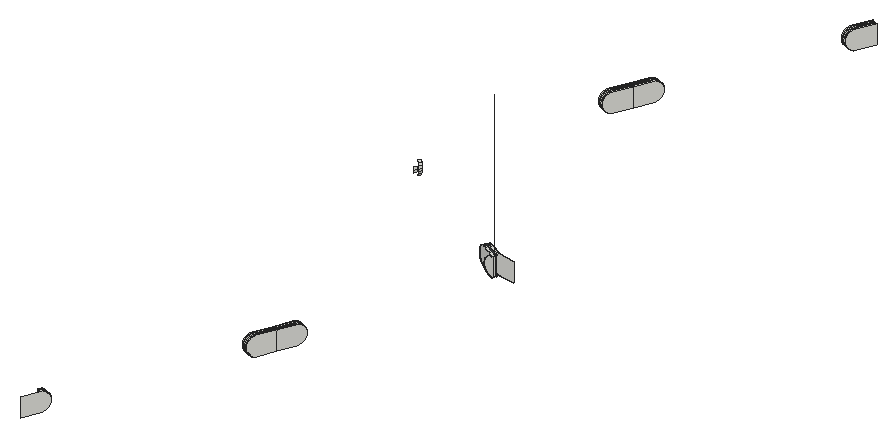
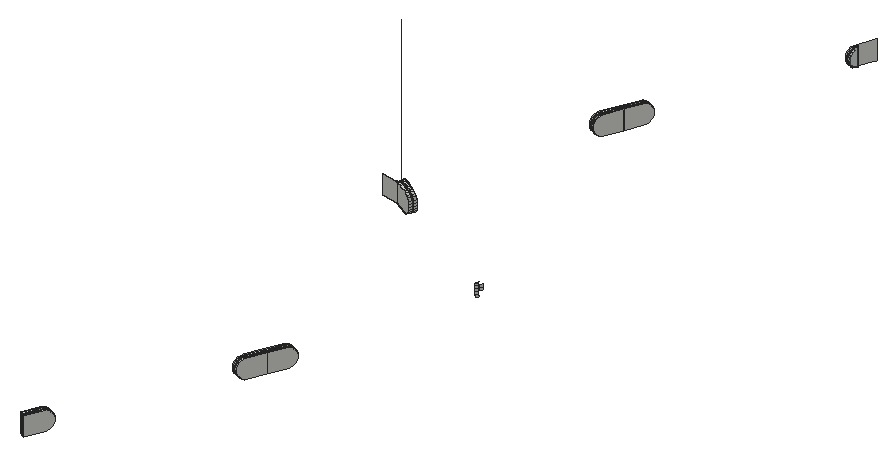
# SketchUp Ruby script. Lengths in inches.
U = 1.inch
M = Sketchup.active_model
def pt(a) = Geom::Point3d.new(a.map { |v| v * U })
def face(e, loops, mat)
  f = e.add_face(loops[0].map { |a| pt(a) })
  loops[1..].each { |l| e.add_face(l.map { |a| pt(a) }).erase! }
  f.material = f.back_material = mat if mat
  f
end
# faces: each face lists its corners as indices into pts; further lists are holes
def faces(e, pts, list, mat = nil) = list.each { |f| face(e, (f[0].is_a?(Array) ? f : [f]).map { |l| l.map { |i| pts[i] } }, mat) }
# xy, xz, yz: faces in a plane at the given z, y or x. An outline is a flat list of corners, or four numbers for a rectangle; further outlines are holes
def ring(l) = l.size == 4 ? [[l[0], l[1]], [l[2], l[1]], [l[2], l[3]], [l[0], l[3]]] : l.each_slice(2).to_a
def flat(e, list, mat, &to3) = list.each { |f| face(e, (f[0].is_a?(Array) ? f : [f]).map { |l| ring(l).map { |u, v| to3.(u, v) } }, mat) }
def xy(e, z, list, mat = nil) = flat(e, list, mat) { |x, y| [x, y, z] }
def xz(e, y, list, mat = nil) = flat(e, list, mat) { |x, z| [x, y, z] }
def yz(e, x, list, mat = nil) = flat(e, list, mat) { |y, z| [x, y, z] }
def lines(e, pts, list) = list.each { |a, b| e.add_line(pt(pts[a]), pt(pts[b])) }
# prism: a flat outline (further loops are holes) pulled along v
def prism(e, loops, v, mat = nil)
  f = face(e, loops, mat); d = Geom::Vector3d.new(v.map { |x| x * U })
  f.pushpull(f.normal.samedirection?(d) ? d.length : -d.length)
end
def box(e, o, s, mat = nil) = prism(e, [[o, [o[0] + s[0], o[1], o[2]], [o[0] + s[0], o[1] + s[1], o[2]], [o[0], o[1] + s[1], o[2]]]], [0, 0, s[2]], mat)
def at(x, y, z, deg = 0) = Geom::Transformation.translation(pt([x, y, z])) * Geom::Transformation.rotation(ORIGIN, Z_AXIS, deg.degrees)
def axes(o, x, y, z) = Geom::Transformation.new([*x, 0, *y, 0, *z, 0, *pt(o).to_a, 1])
def part(name) = M.definitions.add(name)
# library, detail: a bought-in or finely detailed component or shape, given as its bounding box
def library(name, o, s) = part(name).tap { |d| box(d.entities, o, s) }
def detail(e, o, s) = box(e.add_group.entities, o, s)
def put(e, d, t, mat = nil) = e.add_instance(d, t).tap { |i| i.material = mat if mat }
def group(e, t, mat = nil) = e.add_group.tap { |g| g.transformation = t; g.material = mat if mat }.entities
root = M.entities
M.materials.add("Glass_Safety_01").color = [204, 235, 244]
M.materials["Glass_Safety_01"].alpha = 0.1
xy(root,333,[[973.145,833.277,972.892,833.387,972.953,833.526,973.678,835.192,973.931,835.082],[972.711,833.465,972.459,833.576,973.241,835.37,973.496,835.268,972.772,833.605],[973.935,835.091,973.679,835.194,974.413,837.021,974.669,836.918],[973.496,835.268,973.241,835.37,973.245,835.38,973.497,835.27],[973.497,835.27,973.245,835.38,973.975,837.197,974.231,837.094],
  [980.412,857.229,978.702,858.205,978.839,858.444,980.548,857.469,980.545,857.462,980.493,857.47,980.474,857.338],[980.528,857.707,978.936,858.615,979.073,858.855,980.721,857.914,980.561,857.9375],[970.318,886.891,970.065,887.001,970.134,887.159,970.851,888.806,971.104,888.696],[969.884,887.079,969.632,887.189,970.418,888.994,970.671,888.884,969.953,887.238],[971.104,888.696,970.851,888.806,971.637,890.61,971.89,890.5],
  [970.671,888.884,970.418,888.994,971.204,890.799,971.457,890.689],[979.946,908.998,979.693,909.108,979.757,909.255,980.479,910.912,980.732,910.802],[979.513,909.186,979.26,909.296,980.046,911.101,980.299,910.991,979.577,909.334]])
xy(root,333.078,[[973.049,833.748,972.869,833.826,973.496,835.268,973.588,835.231,973.678,835.192],[973.679,835.194,973.588,835.231,973.497,835.27,974.084,836.729,974.267,836.655],[973.588,835.231,973.496,835.268,973.497,835.269,973.497,835.27],[980.548,857.469,979.181,858.249,979.278,858.42,980.63,857.649,980.611,857.652,980.597,857.554],[970.222,887.362,970.042,887.44,970.671,888.884,970.851,888.806],
  [970.851,888.806,970.671,888.884,971.299,890.328,971.48,890.249],[979.85,909.469,979.67,909.547,980.299,910.991,980.479,910.912]],"Glass_Safety_01")
xy(root,335.047,[[973.049,833.748,973.678,835.192,973.588,835.231,973.496,835.268,972.869,833.826],[973.679,835.194,974.267,836.655,974.084,836.729,973.497,835.27,973.588,835.231],[973.588,835.231,973.497,835.27,973.497,835.269,973.496,835.268],[980.548,857.469,980.597,857.554,980.611,857.652,980.63,857.649,979.278,858.42,979.181,858.249],[970.222,887.362,970.851,888.806,970.671,888.884,970.042,887.44],
  [970.851,888.806,971.48,890.249,971.299,890.328,970.671,888.884],[979.85,909.469,980.479,910.912,980.299,910.991,979.67,909.547]],"Glass_Safety_01")
xy(root,335.126,[[973.145,833.277,973.931,835.082,973.678,835.192,972.953,833.526,972.892,833.387],[972.711,833.465,972.772,833.605,973.496,835.268,973.241,835.37,972.459,833.576],[973.935,835.091,974.669,836.918,974.413,837.021,973.679,835.194],[973.496,835.268,973.497,835.27,973.245,835.38,973.241,835.37],[973.497,835.27,974.231,837.094,973.975,837.197,973.245,835.38],
  [980.412,857.229,980.474,857.338,980.493,857.47,980.545,857.462,980.548,857.469,978.839,858.444,978.702,858.205],[980.528,857.707,980.561,857.9375,980.721,857.914,979.073,858.855,978.936,858.615],[970.318,886.891,971.104,888.696,970.851,888.806,970.134,887.159,970.065,887.001],[969.884,887.079,969.953,887.238,970.671,888.884,970.418,888.994,969.632,887.189],[971.104,888.696,971.89,890.5,971.637,890.61,970.851,888.806],
  [970.671,888.884,971.457,890.689,971.204,890.799,970.418,888.994],[979.946,908.998,980.732,910.802,980.479,910.912,979.757,909.255,979.693,909.108],[979.513,909.186,979.577,909.334,980.299,910.991,980.046,911.101,979.26,909.296]])
p = [[963.767,811.746,335.126],[963.765,811.74,335.126],[963.765,811.74,333],[963.767,811.746,333],[963.77,811.753,333],[964.551,813.545,333],
  [964.661,813.797,333.036],[964.763,814.032,333.142],[964.851,814.234,333.311],[964.918,814.389,333.531],[964.961,814.486,333.787],[964.975,814.519,334.0625],
  [964.961,814.486,334.338],[964.918,814.389,334.594],[964.851,814.234,334.814],[964.763,814.032,334.983],[964.661,813.797,335.089],[964.551,813.545,335.126],
  [963.77,811.753,335.126],[964.298,813.655,333],[964.408,813.907,333.036],[964.118,813.733,333],[964.118,813.733,335.126],[964.227,813.986,335.089],
  [964.33,814.221,334.983],[964.418,814.423,334.814],[964.485,814.577,334.594],[964.528,814.675,334.338],[964.542,814.708,334.0625],[964.528,814.675,333.787],
  [964.485,814.577,333.531],[964.418,814.423,333.311],[964.33,814.221,333.142],[964.227,813.986,333.036],[964.298,813.655,335.126],[964.51,814.142,333.142],
  [964.598,814.344,333.311],[964.666,814.499,333.531],[964.708,814.596,333.787],[964.723,814.629,334.0625],[964.708,814.596,334.338],[964.666,814.499,334.594],
  [964.598,814.344,334.814],[964.51,814.142,334.983],[964.408,813.907,335.089],[973.931,835.082,335.126],[973.145,833.277,335.126],[973.035,833.025,335.089],
  [972.932,832.79,334.983],[972.844,832.588,334.814],[972.777,832.433,334.594],[972.735,832.335,334.338],[972.72,832.302,334.0625],[972.735,832.335,333.787],
  [972.777,832.433,333.531],[972.844,832.588,333.311],[972.932,832.79,333.142],[973.035,833.025,333.036],[973.145,833.277,333],[973.931,835.082,333],
  [972.892,833.387,335.126],[972.953,833.526,335.126],[972.953,833.526,333],[972.892,833.387,333],[972.782,833.135,333.036],[972.68,832.9,333.142],
  [972.592,832.698,333.311],[972.524,832.543,333.531],[972.482,832.446,333.787],[972.467,832.412,334.0625],[972.482,832.446,334.338],[972.524,832.543,334.594],
  [972.592,832.698,334.814],[972.68,832.9,334.983],[972.782,833.135,335.089],[972.711,833.465,333],[972.772,833.605,333],[973.496,835.268,333],
  [973.496,835.268,333.078],[973.496,835.268,335.047],[973.496,835.268,335.126],[972.772,833.605,335.126],[972.711,833.465,335.126],[972.602,833.213,335.089],
  [972.499,832.978,334.983],[972.411,832.776,334.814],[972.344,832.621,334.594],[972.301,832.524,334.338],[972.287,832.491,334.0625],[972.301,832.524,333.787],
  [972.344,832.621,333.531],[972.411,832.776,333.311],[972.499,832.978,333.142],[972.602,833.213,333.036],[972.459,833.576,335.126],[973.241,835.37,335.126],
  [973.241,835.37,333],[972.459,833.576,333],[972.349,833.323,333.036],[972.247,833.088,333.142],[972.159,832.886,333.311],[972.091,832.732,333.531],
  [972.049,832.634,333.787],[972.034,832.601,334.0625],[972.049,832.634,334.338],[972.091,832.732,334.594],[972.159,832.886,334.814],[972.247,833.088,334.983],
  [972.349,833.323,335.089],[973.678,835.192,333],[973.678,835.192,335.126],[973.678,835.192,335.047],[973.049,833.748,335.047],[973.049,833.748,333.078],
  [973.678,835.192,333.078],[973.679,835.194,333.078],[973.679,835.194,333],[973.935,835.091,333],[973.935,835.091,335.126],[973.679,835.194,335.126],
  [973.679,835.194,335.047],[974.669,836.918,335.126],[974.669,836.918,333],[974.772,837.173,333.036],[974.867,837.411,333.142],[974.95,837.615,333.311],
  [975.013,837.772,333.531],[975.052,837.87,333.787],[975.066,837.904,334.0625],[975.052,837.87,334.338],[975.013,837.772,334.594],[974.95,837.615,334.814],
  [974.867,837.411,334.983],[974.772,837.173,335.089],[974.413,837.021,335.126],[974.413,837.021,333],[974.267,836.655,333.078],[974.267,836.655,335.047],
  [973.497,835.27,333.078],[973.497,835.27,333],[973.245,835.38,333],[973.245,835.38,335.126],[973.497,835.27,335.126],[973.497,835.27,335.047],
  [974.231,837.094,333],[974.333,837.349,333.036],[974.429,837.587,333.142],[974.511,837.791,333.311],[974.574,837.948,333.531],[974.614,838.047,333.787],
  [974.627,838.08,334.0625],[974.614,838.047,334.338],[974.574,837.948,334.594],[974.511,837.791,334.814],[974.429,837.587,334.983],[974.333,837.349,335.089],
  [974.231,837.094,335.126],[973.243,835.375,333],[973.243,835.375,335.126],[973.975,837.197,335.126],[974.078,837.452,335.089],[974.173,837.69,334.983],
  [974.256,837.894,334.814],[974.319,838.051,334.594],[974.358,838.149,334.338],[974.372,838.183,334.0625],[974.358,838.149,333.787],[974.319,838.051,333.531],
  [974.256,837.894,333.311],[974.173,837.69,333.142],[974.078,837.452,333.036],[973.975,837.197,333],[974.516,837.276,333.036],[974.612,837.514,333.142],
  [974.694,837.718,333.311],[974.757,837.875,333.531],[974.797,837.973,333.787],[974.81,838.007,334.0625],[974.797,837.973,334.338],[974.757,837.875,334.594],
  [974.694,837.718,334.814],[974.612,837.514,334.983],[974.516,837.276,335.089],[980.412,857.229,335.126],[978.702,858.205,335.126],[978.463,858.341,335.089],
  [978.24,858.468,334.983],[978.049,858.578,334.814],[977.902,858.661,334.594],[977.81,858.714,334.338],[977.779,858.732,334.0625],[977.81,858.714,333.787],
  [977.902,858.661,333.531],[978.049,858.578,333.311],[978.24,858.468,333.142],[978.463,858.341,333.036],[978.702,858.205,333],[980.412,857.229,333],
  [980.453,857.197,333],[980.543,857.184,333],[980.543,857.184,335.126],[980.453,857.197,335.126],[980.181,857.237,335.089],[979.927,857.274,334.983],
  [979.709,857.306,334.814],[979.542,857.33,334.594],[979.437,857.345,334.338],[979.401,857.351,334.0625],[979.437,857.345,333.787],[979.542,857.33,333.531],
  [979.709,857.306,333.311],[979.927,857.274,333.142],[980.181,857.237,333.036],[979.967,857.547,333.142],[980.221,857.51,333.036],[980.489,857.471,333],
  [980.493,857.47,333],[980.474,857.338,333],[980.548,857.469,333],[978.839,858.444,333],[978.839,858.444,335.126],[980.548,857.469,335.126],
  [980.548,857.469,335.047],[979.181,858.249,335.047],[979.181,858.249,333.078],[980.548,857.469,333.078],[980.221,857.51,335.089],[980.489,857.471,335.125],
  [979.749,857.578,333.311],[979.582,857.603,333.531],[979.477,857.618,333.787],[979.441,857.623,334.0625],[979.477,857.618,334.338],[979.582,857.603,334.594],
  [979.749,857.578,334.814],[979.967,857.547,334.983],[980.493,857.47,335.126],[980.528,857.707,335.126],[978.936,858.615,335.126],[978.936,858.615,333],
  [980.528,857.707,333],[980.63,857.649,333],[980.646,857.64,333],[980.646,857.64,333.078],[980.63,857.649,333.078],[979.278,858.42,333.078],
  [979.278,858.42,335.047],[980.63,857.649,335.047],[980.646,857.64,335.047],[980.646,857.64,335.126],[980.63,857.649,335.126],[980.249,857.704,333.036],
  [980.517,857.665,333],[980.517,857.665,335.125],[980.249,857.704,335.089],[979.996,857.741,334.983],[979.778,857.773,334.814],[979.611,857.798,334.594],
  [979.505,857.813,334.338],[979.47,857.818,334.0625],[979.505,857.813,333.787],[979.611,857.798,333.531],[979.778,857.773,333.311],[979.996,857.741,333.142],
  [980.721,857.914,335.126],[982.509,857.653,335.126],[982.509,857.653,333],[980.721,857.914,333],[980.561,857.9375,333],[980.289,857.977,333.036],
  [980.035,858.014,333.142],[979.817,858.046,333.311],[979.65,858.07,333.531],[979.545,858.086,333.787],[979.509,858.091,334.0625],[979.545,858.086,334.338],
  [979.65,858.07,334.594],[979.817,858.046,334.814],[980.035,858.014,334.983],[980.289,857.977,335.089],[980.561,857.9375,335.126],[980.521,857.665,333],
  [980.782,857.879,335.126],[980.782,857.879,333],[979.073,858.855,333],[978.834,858.991,333.036],[978.611,859.118,333.142],[978.42,859.227,333.311],
  [978.273,859.311,333.531],[978.181,859.364,333.787],[978.149,859.382,334.0625],[978.181,859.364,334.338],[978.273,859.311,334.594],[978.42,859.227,334.814],
  [978.611,859.118,334.983],[978.834,858.991,335.089],[979.073,858.855,335.126],[978.6,858.581,333.036],[978.377,858.708,333.142],[978.6,858.581,335.089],
  [978.377,858.708,334.983],[978.186,858.817,334.814],[978.039,858.901,334.594],[977.947,858.953,334.338],[977.915,858.971,334.0625],[977.947,858.953,333.787],
  [978.039,858.901,333.531],[978.186,858.817,333.311],[978.697,858.752,333.036],[978.475,858.879,333.142],[978.283,858.988,333.311],[978.137,859.072,333.531],
  [978.044,859.124,333.787],[978.013,859.142,334.0625],[978.044,859.124,334.338],[978.137,859.072,334.594],[978.283,858.988,334.814],[978.475,858.879,334.983],
  [978.697,858.752,335.089],[971.104,888.696,335.126],[970.318,886.891,335.126],[970.208,886.639,335.089],[970.105,886.403,334.983],[970.017,886.202,334.814],
  [969.95,886.047,334.594],[969.908,885.949,334.338],[969.893,885.916,334.0625],[969.908,885.949,333.787],[969.95,886.047,333.531],[970.017,886.202,333.311],
  [970.105,886.403,333.142],[970.208,886.639,333.036],[970.318,886.891,333],[971.104,888.696,333],[970.065,887.001,335.126],[970.134,887.159,335.126],
  [970.134,887.159,333],[970.065,887.001,333],[969.955,886.749,333.036],[969.853,886.514,333.142],[969.765,886.312,333.311],[969.697,886.157,333.531],
  [969.655,886.059,333.787],[969.641,886.026,334.0625],[969.655,886.059,334.338],[969.697,886.157,334.594],[969.765,886.312,334.814],[969.853,886.514,334.983],
  [969.955,886.749,335.089],[969.884,887.079,333],[969.953,887.238,333],[969.953,887.238,335.126],[969.884,887.079,335.126],[969.775,886.827,335.089],
  [969.672,886.592,334.983],[969.584,886.39,334.814],[969.517,886.235,334.594],[969.474,886.138,334.338],[969.46,886.105,334.0625],[969.474,886.138,333.787],
  [969.517,886.235,333.531],[969.584,886.39,333.311],[969.672,886.592,333.142],[969.775,886.827,333.036],[969.632,887.189,335.126],[970.418,888.994,335.126],
  [970.418,888.994,333],[969.632,887.189,333],[969.522,886.937,333.036],[969.42,886.702,333.142],[969.332,886.5,333.311],[969.264,886.345,333.531],
  [969.222,886.248,333.787],[969.207,886.215,334.0625],[969.222,886.248,334.338],[969.264,886.345,334.594],[969.332,886.5,334.814],[969.42,886.702,334.983],
  [969.522,886.937,335.089],[970.671,888.884,335.126],[970.671,888.884,333],[970.671,888.884,333.078],[970.042,887.44,333.078],[970.042,887.44,335.047],
  [970.671,888.884,335.047],[970.851,888.806,333],[970.851,888.806,335.126],[970.851,888.806,335.047],[970.222,887.362,335.047],[970.222,887.362,333.078],
  [970.851,888.806,333.078],[971.89,890.5,335.126],[971.89,890.5,333],[972,890.753,333.036],[972.102,890.988,333.142],[972.19,891.189,333.311],
  [972.257,891.344,333.531],[972.3,891.442,333.787],[972.314,891.475,334.0625],[972.3,891.442,334.338],[972.257,891.344,334.594],[972.19,891.189,334.814],
  [972.102,890.988,334.983],[972,890.753,335.089],[971.637,890.61,335.126],[971.637,890.61,333],[971.48,890.249,333.078],[971.48,890.249,335.047],
  [971.457,890.689,333],[971.457,890.689,335.126],[971.299,890.328,335.047],[971.299,890.328,333.078],[971.204,890.799,335.126],[971.314,891.051,335.089],
  [971.416,891.286,334.983],[971.504,891.488,334.814],[971.571,891.643,334.594],[971.614,891.74,334.338],[971.628,891.774,334.0625],[971.614,891.74,333.787],
  [971.571,891.643,333.531],[971.504,891.488,333.311],[971.416,891.286,333.142],[971.314,891.051,333.036],[971.204,890.799,333],[971.747,890.863,333.036],
  [971.849,891.098,333.142],[971.937,891.299,333.311],[972.005,891.454,333.531],[972.047,891.552,333.787],[972.061,891.585,334.0625],[972.047,891.552,334.338],
  [972.005,891.454,334.594],[971.937,891.299,334.814],[971.849,891.098,334.983],[971.747,890.863,335.089],[971.566,890.941,333.036],[971.566,890.941,335.089],
  [971.669,891.176,334.983],[971.757,891.378,334.814],[971.824,891.533,334.594],[971.867,891.63,334.338],[971.881,891.663,334.0625],[971.867,891.63,333.787],
  [971.824,891.533,333.531],[971.757,891.378,333.311],[971.669,891.176,333.142],[980.732,910.802,335.126],[979.946,908.998,335.126],[979.836,908.745,335.089],
  [979.734,908.51,334.983],[979.646,908.308,334.814],[979.578,908.154,334.594],[979.536,908.056,334.338],[979.521,908.023,334.0625],[979.536,908.056,333.787],
  [979.578,908.154,333.531],[979.646,908.308,333.311],[979.734,908.51,333.142],[979.836,908.745,333.036],[979.946,908.998,333],[980.732,910.802,333],
  [979.693,909.108,335.126],[979.757,909.255,335.126],[979.757,909.255,333],[979.693,909.108,333],[979.583,908.855,333.036],[979.481,908.62,333.142],
  [979.393,908.418,333.311],[979.326,908.264,333.531],[979.283,908.166,333.787],[979.269,908.133,334.0625],[979.283,908.166,334.338],[979.326,908.264,334.594],
  [979.393,908.418,334.814],[979.481,908.62,334.983],[979.583,908.855,335.089],[979.513,909.186,333],[979.577,909.334,333],[979.577,909.334,335.126],
  [979.513,909.186,335.126],[979.403,908.934,335.089],[979.3,908.699,334.983],[979.213,908.497,334.814],[979.145,908.342,334.594],[979.103,908.245,334.338],
  [979.088,908.212,334.0625],[979.103,908.245,333.787],[979.145,908.342,333.531],[979.213,908.497,333.311],[979.3,908.699,333.142],[979.403,908.934,333.036],
  [979.26,909.296,335.126],[980.046,911.101,335.126],[980.046,911.101,333],[979.26,909.296,333],[979.15,909.044,333.036],[979.048,908.809,333.142],
  [978.96,908.607,333.311],[978.892,908.452,333.531],[978.85,908.355,333.787],[978.836,908.322,334.0625],[978.85,908.355,334.338],[978.892,908.452,334.594],
  [978.96,908.607,334.814],[979.048,908.809,334.983],[979.15,909.044,335.089],[980.299,910.991,335.126],[980.299,910.991,333],[980.299,910.991,333.078],
  [979.67,909.547,333.078],[979.67,909.547,335.047],[980.299,910.991,335.047],[980.479,910.912,333],[980.479,910.912,335.126],[980.479,910.912,335.047],
  [979.85,909.469,335.047],[979.85,909.469,333.078],[980.479,910.912,333.078],[972.869,833.826,335.047],[972.869,833.826,333.078],[973.588,835.231,333.078],
  [973.588,835.231,335.047],[973.497,835.269,335.047],[973.497,835.269,333.078],[974.084,836.729,333.078],[974.084,836.729,335.047],[964.165,814.533,333.311],
  [964.232,814.6875,333.531],[964.361,866.932,333.531],[964.215,867.016,333.311],[964.351,867.255,333.311],[964.498,867.171,333.531],[964.275,814.785,333.787],
  [964.454,866.879,333.787],[964.59,867.119,333.787],[964.289,814.818,334.0625],[964.356,866.708,333.787],[964.388,866.69,334.0625],[964.251,866.451,334.0625],
  [964.22,866.469,333.787],[964.485,866.861,334.0625],[964.622,867.101,334.0625],[964.275,814.785,334.338],[964.356,866.708,334.338],[964.22,866.469,334.338],
  [964.454,866.879,334.338],[964.59,867.119,334.338],[964.232,814.6875,334.594],[964.361,866.932,334.594],[964.498,867.171,334.594],[964.165,814.533,334.814],
  [964.215,867.016,334.814],[964.351,867.255,334.814],[964.077,814.331,334.983],[980.474,857.338,335.126],[980.493,857.47,351.283],[980.489,857.471,351.284],
  [980.521,857.665,335.126]]
faces(root,p,[[0,1,2,3,4,5,6,7,8,9,10,11,12,13,14,15,16,17,18],[19,20,6,5],[20,35,7,6],[45,46,47,48,49,50,51,52,53,54,55,56,57,58,59],[60,61,62,63,64,65,66,67,68,69,70,71,72,73,74],[75,76,77,78,79,80,81,82,83,84,85,86,87,88,89,90,91,92,93],[94,95,96,97,98,99,100,101,102,103,104,105,106,107,108],[65,64,57,56],
  [93,92,99,98],[64,63,58,57],[75,93,98,97],[109,62,61,110,111,112,113,114],[109,114,111,110,45,59],[115,116,117,118,119,120],[121,118,117,122,123,124,125,126,127,128,129,130,131,132,133],[119,134,135,116,115,136,137,120],
  [77,78,79,80,95,96],[138,139,140,141,142,143],[142,80,79,78,77,139,138,143],[142,80,79,78,77,139,144,145,146,147,148,149,150,151,152,153,154,155,156],[157,96,95,158,141,140],[95,158,141,159,160,161,162,163,164,165,166,167,168,169,170,171,140,157,96],[135,172,123,122],[145,144,171,170],
  [172,173,124,123],[146,145,170,169],[183,184,185,186,187,188,189,190,191,192,193,194,195,196,197],[198,199,200,201,202,203,204,205,206,207,208,209,210,211,212],[213,214,212,211],[214,215,216,217,198,212],[218,219,220,221,222,223,224,225],[226,227,215,214,213,228,229,230,231,232,233,234,235],
  [237,238,239,240,241,242,243,244,245,246,247,248,249,250],[251,252,253,254,255,256,257,258,259,260,261,262,263],[264,265,266,267,268,269,270,271,272,273,274,275,276,277,278,279,280],[251,263,270,269],[252,251,269,268,240,281],[264,282,283,267,284,285,286,287,288,289,290,291,292,293,294,295,296],[297,219,196,195],[298,297,195,194],
  [239,308,285,284],[308,309,286,285],[319,320,321,322,323,324,325,326,327,328,329,330,331,332,333],[334,335,336,337,338,339,340,341,342,343,344,345,346,347,348],[349,350,351,352,353,354,355,356,357,358,359,360,361,362,363],[364,365,366,367,368,369,370,371,372,373,374,375,376,377,378],[339,338,331,330],[363,362,369,368],
  [338,337,332,331],[349,363,368,367],[379,351,350,380,381,382,383,384],[385,336,335,386,387,388,389,390],[385,390,387,386,319,333],[391,319,333,392,393,394,395,396,397,398,399,400,401,402,403],[386,404,405,385,390,406,407,387],[381,380,366,365,379,384],
  [380,408,409,379,384,410,411,381],[365,412,413,414,415,416,417,418,419,420,421,422,423,424,366],[405,425,393,392],[436,408,424,423],[425,426,394,393],[446,436,423,422],[447,448,449,450,451,452,453,454,455,456,457,458,459,460,461],[462,463,464,465,466,467,468,469,470,471,472,473,474,475,476],
  [477,478,479,480,481,482,483,484,485,486,487,488,489,490,491],[492,493,494,495,496,497,498,499,500,501,502,503,504,505,506],[467,466,459,458],[491,490,497,496],[466,465,460,459],[477,491,496,495],[507,479,478,508,509,510,511,512],[513,464,463,514,515,516,517,518],
  [509,508,494,493,507,512],[35,36,8,7],[66,65,56,55],[92,91,100,99],[173,174,125,124],[147,146,169,168],[228,213,211,210],[263,262,271,270],
  [307,298,194,193],[309,310,287,286],[340,339,330,329],[362,361,370,369],[426,427,395,394],[445,446,422,421],[468,467,458,457],[490,489,498,497],
  [36,37,9,8],[30,31,527,528],[67,66,55,54],[91,90,101,100],[174,175,126,125],[148,147,168,167],[229,228,210,209],[262,261,272,271],
  [306,307,193,192],[310,311,288,287],[529,530,531,532],[341,340,329,328],[361,360,371,370],[427,428,396,395],[444,445,421,420],[469,468,457,456],
  [489,488,499,498],[37,38,10,9],[29,30,528,533],[68,67,54,53],[90,89,102,101],[175,176,127,126],[149,148,167,166],[230,229,209,208],
  [261,260,273,272],[305,306,192,191],[311,312,289,288],[534,529,532,535],[342,341,328,327],[360,359,372,371],[428,429,397,396],[443,444,420,419],
  [470,469,456,455],[488,487,500,499],[38,39,11,10],[28,29,533,536],[69,68,53,52],[89,88,103,102],[176,177,128,127],[150,149,166,165],
  [231,230,208,207],[260,259,274,273],[304,305,191,190],[312,313,290,289],[537,538,539,540],[541,534,535,542],[343,342,327,326],[359,358,373,372],
  [429,430,398,397],[442,443,419,418],[471,470,455,454],[487,486,501,500],[39,40,12,11],[27,28,536,543],[70,69,52,51],[88,87,104,103],
  [177,178,129,128],[151,150,165,164],[232,231,207,206],[259,258,275,274],[303,304,190,189],[313,314,291,290],[538,544,545,539],[546,541,542,547],
  [344,343,326,325],[358,357,374,373],[430,431,399,398],[441,442,418,417],[472,471,454,453],[486,485,502,501],[40,41,13,12],[26,27,543,548],
  [71,70,51,50],[87,86,105,104],[178,179,130,129],[152,151,164,163],[233,232,206,205],[258,257,276,275],[302,303,189,188],[314,315,292,291],
  [549,546,547,550],[345,344,325,324],[357,356,375,374],[431,432,400,399],[440,441,417,416],[473,472,453,452],[485,484,503,502],[41,42,14,13],
  [25,26,548,551],[72,71,50,49],[86,85,106,105],[179,180,131,130],[153,152,163,162],[234,233,205,204],[257,256,277,276],[301,302,188,187],
  [315,316,293,292],[552,549,550,553],[346,345,324,323],[356,355,376,375],[432,433,401,400],[439,440,416,415],[474,473,452,451],[484,483,504,503],
  [42,43,15,14],[24,25,551,554],[73,72,49,48],[85,84,107,106],[180,181,132,131],[154,153,162,161],[235,234,204,203],[256,255,278,277],
  [300,301,187,186],[316,317,294,293],[347,346,323,322],[355,354,377,376],[433,434,402,401],[438,439,415,414],[475,474,451,450],[483,482,505,504],
  [43,44,16,15],[74,73,48,47],[84,83,108,107],[181,182,133,132],[155,154,161,160],[226,235,203,202],[255,254,279,278],[299,300,186,185],
  [317,318,295,294],[348,347,322,321],[354,353,378,377],[434,435,403,402],[437,438,414,413],[476,475,450,449],[482,481,506,505],[44,34,17,16],
  [60,74,47,46],[83,82,94,108],[182,134,121,133],[156,155,160,159],[236,227,226,202,201,555],[253,558,237,280,279,254],[220,299,185,184],[318,238,296,295],
  [334,348,321,320],[353,352,364,378],[435,404,391,403],[409,437,413,412],[462,476,449,448],[481,480,492,506]])
faces(root,p,[[21,22,23,24,25,26,27,28,29,30,31,32,33],[34,19,20,35,36,37,38,39,40,41,42,43,44],[134,135,172,173,174,175,176,177,178,179,180,181,182],[144,156,155,154,153,152,151,150,149,148,147,146,145],[227,215,216,236],[219,220,299,300,301,302,303,304,305,306,307,298,297],[238,239,308,309,310,311,312,313,314,315,316,317,318],[404,405,425,426,427,428,429,430,431,432,433,434,435],
  [408,409,437,438,439,440,441,442,443,444,445,446,436],[113,112,519,520],[114,113,112,111],[519,79,78,520],[521,522,79,78],[143,522,521,138],[114,521,522,111],[522,521,115,120],
  [136,115,120,137],[523,143,138,524,78,79],[525,138,143,526],[136,525,526,137],[225,224,223,222],[244,243,248,247,246,245],[223,246,245,224],[389,388,383,382],
  [382,381,384,383],[390,389,388,387],[384,387,390,381],[406,390,387,407],[381,411,410,384],[407,406,411,410],[517,516,511,510],[510,509,512,511],
  [518,517,516,515],[512,515,518,509],[227,556,557],[556,227,236]],"Glass_Safety_01")
